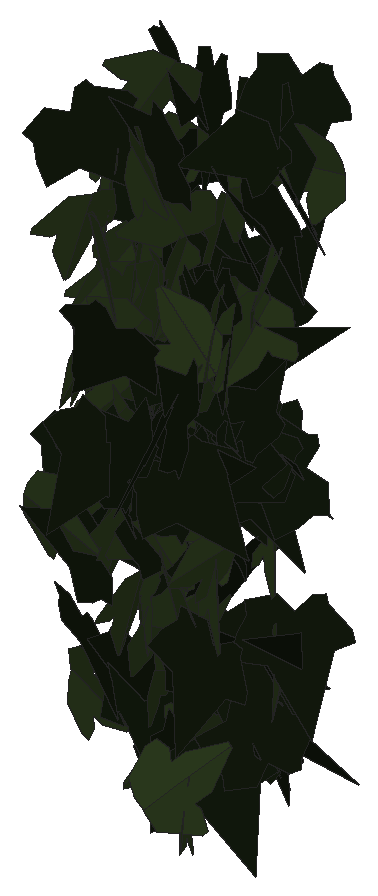
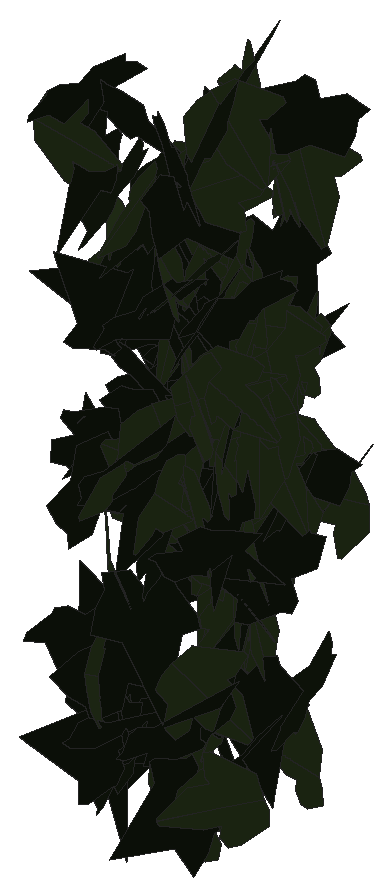
# SketchUp Ruby script. Lengths in inches.
U = 1.inch
M = Sketchup.active_model
def pt(a) = Geom::Point3d.new(a.map { |v| v * U })
def face(e, loops, mat)
  f = e.add_face(loops[0].map { |a| pt(a) })
  loops[1..].each { |l| e.add_face(l.map { |a| pt(a) }).erase! }
  f.material = f.back_material = mat if mat
  f
end
# faces: each face lists its corners as indices into pts; further lists are holes
def faces(e, pts, list, mat = nil) = list.each { |f| face(e, (f[0].is_a?(Array) ? f : [f]).map { |l| l.map { |i| pts[i] } }, mat) }
# xy, xz, yz: faces in a plane at the given z, y or x. An outline is a flat list of corners, or four numbers for a rectangle; further outlines are holes
def ring(l) = l.size == 4 ? [[l[0], l[1]], [l[2], l[1]], [l[2], l[3]], [l[0], l[3]]] : l.each_slice(2).to_a
def flat(e, list, mat, &to3) = list.each { |f| face(e, (f[0].is_a?(Array) ? f : [f]).map { |l| ring(l).map { |u, v| to3.(u, v) } }, mat) }
def xy(e, z, list, mat = nil) = flat(e, list, mat) { |x, y| [x, y, z] }
def xz(e, y, list, mat = nil) = flat(e, list, mat) { |x, z| [x, y, z] }
def yz(e, x, list, mat = nil) = flat(e, list, mat) { |y, z| [x, y, z] }
def lines(e, pts, list) = list.each { |a, b| e.add_line(pt(pts[a]), pt(pts[b])) }
# prism: a flat outline (further loops are holes) pulled along v
def prism(e, loops, v, mat = nil)
  f = face(e, loops, mat); d = Geom::Vector3d.new(v.map { |x| x * U })
  f.pushpull(f.normal.samedirection?(d) ? d.length : -d.length)
end
def box(e, o, s, mat = nil) = prism(e, [[o, [o[0] + s[0], o[1], o[2]], [o[0] + s[0], o[1] + s[1], o[2]], [o[0], o[1] + s[1], o[2]]]], [0, 0, s[2]], mat)
def at(x, y, z, deg = 0) = Geom::Transformation.translation(pt([x, y, z])) * Geom::Transformation.rotation(ORIGIN, Z_AXIS, deg.degrees)
def axes(o, x, y, z) = Geom::Transformation.new([*x, 0, *y, 0, *z, 0, *pt(o).to_a, 1])
def part(name) = M.definitions.add(name)
# library, detail: a bought-in or finely detailed component or shape, given as its bounding box
def library(name, o, s) = part(name).tap { |d| box(d.entities, o, s) }
def detail(e, o, s) = box(e.add_group.entities, o, s)
def put(e, d, t, mat = nil) = e.add_instance(d, t).tap { |i| i.material = mat if mat }
def group(e, t, mat = nil) = e.add_group.tap { |g| g.transformation = t; g.material = mat if mat }.entities
root = M.entities
M.materials.add("efeu1").color = [18, 25, 13]
M.materials.add("efeu2").color = [43, 57, 29]
c1 = part("ivyleaf_10")
p = [[0,0.5,-0.03],[-0.0625,2.02,-0.43],[-0.19,2.01,-0.46],[-0.54,1.05,-0.29],[-0.52,0.625,-0.18],[-0.83,0.76,-0.28],
  [-1.16,0.64,-0.33],[-1.15,0.33,-0.24],[-0.77,-0.39,0.02],[-0.3,-0.51,0.16],[0.04,-0.48,0.23],[-0.02,2.01,-0.4375],
  [-0.06,2.01,-0.43],[0.04,-0.49,0.23],[0.67,-0.49,0.14],[1.38,0.36,-0.2],[1.375,0.51,-0.24],[0.81,0.65,-0.19],
  [0.62,0.59,-0.15],[0.6,1.09,-0.28],[0.5,1.23,-0.31]]
faces(c1.entities,p,[[0,1,2,3,4,5,6,7,8,9,10],[11,12,0,13,14,15,16,17,18,19,20]],"efeu2")
c2 = part("ivyleaf_9")
p = [[1.54,2.16,1.25],[1.36,2.04,1.19],[-0.21,0.99,0.68],[-0.71,1.11,0.82],[-0.85,0.86,0.67],[-0.8,0.17,0.21],
  [-0.9,-0.01,0.1],[-0.67,-0.16,-0.02],[-0.08,-0.08,-0.05],[-0.03,-0.6,-0.4],[0.65,-0.88,-0.66],[0.83,-0.6,-0.49],
  [1.29,-0.42,-0.43],[1.8125,-0.07,-0.26],[1.21,0.44,0.15]]
faces(c2.entities,p,[[0,1,2,3,4,5,6,7,8,9,10,11,12,13,14]],"efeu1")
put(root,c1,axes([29.63,222.12,219.35],[-0.26898,0.10914,-0.40711],[0.32327,-0.25646,-0.28235],[-0.27045,-0.41511,0.0674]))
put(root,c1,axes([30.23,221.64,218.46],[-0.36147,-0.05554,0.34097],[-0.33899,-0.03802,-0.36557],[0.06653,-0.49545,-0.01017]))
put(root,c1,axes([30.02,221.95,220.1],[-0.21554,-0.44343,0.08317],[-0.02161,-0.08192,-0.49277],[0.45064,-0.21602,0.01615]))
put(root,c2,axes([29.64,221.65,215.46],[0.22446,-0.38681,0.2236],[0.09963,-0.20059,-0.44703],[0.43554,0.24524,-0.01298]))
put(root,c1,axes([30,222.03,220.38],[0.07333,0.24047,-0.4322],[-0.16199,-0.40115,-0.25068],[-0.46731,0.17679,0.01908]))
put(root,c1,axes([29.57,221.67,214.59],[0.03065,-0.04016,0.49744],[0.49615,-0.05127,-0.03471],[0.0538,0.49574,0.03671]))
put(root,c1,axes([30.24,222.63,219.8125],[0.27612,0.06542,-0.41168],[-0.41684,0.04646,-0.27219],[0.00264,0.49352,0.08019]))
put(root,c2,axes([29.82,222.73,221.03],[-0.04323,-0.48304,-0.12167],[0.01583,0.12073,-0.48495],[0.49788,-0.04578,0.00485]))
put(root,c1,axes([30.1,221.95,218.91],[-0.34806,-0.35895,0.00311],[-0.00149,-0.00289,-0.49999],[0.35896,-0.34806,0.00094]))
put(root,c1,axes([30.17,221.73,218.73],[-0.01748,-0.22838,0.44445],[-0.04716,-0.44199,-0.22896],[0.49746,-0.04992,-0.00609]))
put(root,c1,axes([30.33,222.75,219.53],[0.01714,0.13451,0.48126],[-0.20471,-0.4374,0.12954],[0.45585,-0.20148,0.04007]))
put(root,c1,axes([30.24,222.03,220.47],[-0.45318,0.19204,0.08801],[-0.07981,0.03721,-0.49218],[-0.19559,-0.46015,-0.00308]))
put(root,c1,axes([29.82,220.66,217.52],[-0.12335,0.05379,-0.48155],[0.44157,-0.19212,-0.13456],[-0.19951,-0.45847,-0.00011]))
put(root,c2,axes([29.91,221.32,218.38],[0.00236,-0.24218,-0.43743],[0.18486,0.40686,-0.22426],[0.46457,-0.16067,0.09145]))
put(root,c2,axes([30.36,222.92,217.68],[-0.38535,-0.27616,0.15887],[-0.1233,-0.10063,-0.47399],[0.29377,-0.40449,0.00945]))
put(root,c1,axes([30.05,222.625,218.82],[0.13286,-0.31833,0.36196],[0.24291,-0.28008,-0.33548],[0.41634,0.26499,0.08023]))
put(root,c2,axes([30.31,222.17,219.47],[0.29122,-0.07064,-0.40025],[-0.38944,0.0924,-0.29966],[0.1163,0.48628,-0.0012]))
put(root,c2,axes([29.97,221.62,216.92],[0.08087,0.03347,0.49228],[0.45491,0.18814,-0.08753],[-0.19109,0.46204,-0.00002]))
put(root,c1,axes([30.29,221.73,217.45],[0.13576,-0.4812,0.00356],[0.00097,-0.00342,-0.49999],[0.48121,0.13577,0]))
put(root,c1,axes([30.08,221.4375,217.75],[-0.20876,-0.15927,-0.4255],[0.3328,0.26517,-0.26254],[0.30929,-0.39283,-0.0047]))
put(root,c1,axes([30.55,221.54,219.77],[-0.36925,-0.1456,0.30406],[-0.27135,-0.13924,-0.39621],[0.20005,-0.45761,0.02381]))
put(root,c1,axes([30.11,221.11,219.5],[0.0309,-0.05768,0.4957],[0.28165,-0.40798,-0.06503],[0.41197,0.28325,0.00728]))
put(root,c2,axes([30.07,220.95,222.72],[0.01722,-0.20561,-0.45544],[0.107,0.44666,-0.19759],[0.48811,-0.09066,0.05939]))
put(root,c2,axes([30.34,221,216.88],[0.15048,-0.47353,-0.05592],[0.0275,-0.04993,0.49674],[-0.47603,-0.15257,0.01102]))
put(root,c2,axes([30.15,223,220.64],[0.01103,-0.39511,0.30622],[-0.00501,-0.30636,-0.39512],[0.49985,0.00565,-0.01072]))
put(root,c1,axes([29.98,222.39,214.33],[0.11317,0.08031,0.48036],[0.34727,0.33246,-0.13739],[-0.34146,0.36472,0.01947]))
put(root,c2,axes([30,221.53,217.92],[0.20469,-0.34611,0.29718],[0.13944,-0.26267,-0.40195],[0.43435,0.24742,-0.01101]))
put(root,c1,axes([30.15,221.52,222.07],[0.34931,-0.26102,0.24465],[0.20487,-0.13436,-0.43586],[0.29328,0.40474,0.01309]))
put(root,c1,axes([30.52,222.1,222.94],[-0.28599,-0.32336,0.25228],[-0.16848,-0.18778,-0.43168],[0.37393,-0.33192,-0.00155]))
put(root,c2,axes([30.44,222.08,218.18],[0.33035,0.04369,-0.37277],[-0.37394,-0.00436,-0.33189],[-0.03226,0.49807,0.0298]))
put(root,c1,axes([30.42,220.72,221.69],[-0.11695,-0.47986,0.07786],[-0.01615,-0.0762,-0.4939],[0.48586,-0.11804,0.00232]))
put(root,c1,axes([30.6,222.6,215.77],[-0.21113,-0.28887,0.34926],[-0.20553,-0.28238,-0.3578],[0.40396,-0.29465,0.00049]))
put(root,c2,axes([30.52,221.61,215.38],[0.25137,0.25331,-0.35022],[-0.25309,-0.24215,-0.3568],[-0.35037,0.35665,0.00648]))
put(root,c1,axes([30.31,222.7,219.15],[0.32938,-0.37434,-0.03713],[0.02483,-0.02761,0.49862],[-0.37536,-0.33031,0.0004]))
put(root,c1,axes([30.44,221.42,217.2],[0.05093,-0.47747,0.13939],[0.02894,-0.13703,-0.47998],[0.49656,0.05696,0.01368]))
put(root,c1,axes([30.75,222.13,221.93],[-0.15932,-0.04876,-0.47142],[-0.43701,-0.17736,0.16604],[-0.18342,0.46493,0.0139]))
put(root,c1,axes([30.41,221.96,220.99],[-0.06647,0.36301,-0.33736],[0.0188,-0.33828,-0.36771],[-0.49521,-0.06156,0.03132]))
put(root,c2,axes([30.3,222,214.65],[0.1057,-0.48864,-0.00758],[-0.00159,0.00741,-0.49994],[0.4887,0.10571,0.00002]))
put(root,c1,axes([30.57,221.47,216.35],[0.05701,-0.49648,0.0162],[0.00135,-0.01615,-0.49974],[0.49674,0.05702,-0.0005]))
put(root,c2,axes([30.34,222.64,222.69],[0.03214,-0.28726,0.40798],[0.11451,-0.39367,-0.2862],[0.48565,0.11183,0.04048]))
put(root,c2,axes([30.68,222.25,215.22],[0.27303,-0.35536,0.22176],[-0.12425,0.18408,0.44797],[-0.40002,-0.29972,0.01221]))
put(root,c1,axes([30.52,221.57,220.01],[-0.45121,0.02215,0.21428],[0.21421,-0.00661,0.45174],[0.02284,0.49947,-0.00352]))
put(root,c1,axes([30.74,222.33,213.88],[0.00643,-0.08137,0.49329],[-0.0088,-0.49328,-0.08125],[0.49988,-0.00764,-0.00777]))
put(root,c1,axes([30.81,222.3,218.07],[0.32473,-0.29879,-0.2351],[-0.1473,0.18616,-0.44005],[0.3505,0.35506,0.03289]))
put(root,c1,axes([30.77,221.64,215.21],[0.0811,-0.22392,-0.43964],[-0.03764,0.44143,-0.23178],[0.49194,0.07069,0.05475]))
put(root,c2,axes([30.96,222.8,214.84],[-0.25328,-0.4306,-0.02069],[-0.00709,-0.01983,0.49956],[-0.43104,0.25335,0.00394]))
put(root,c1,axes([30.625,222.51,219.55],[0.34826,-0.30325,0.1917],[0.14008,-0.13103,-0.46175],[0.33029,0.37532,-0.00631]))
put(root,c2,axes([31.1,221.75,217.01],[-0.35783,0.30321,0.17327],[-0.13687,0.10647,-0.46897],[-0.32129,-0.38305,0.00681]))
put(root,c2,axes([30.89,221.57,217.01],[-0.10067,-0.41188,0.26498],[0.0895,0.2505,0.42337],[-0.48151,0.13267,0.02329]))
put(root,c2,axes([30.81,222.27,214.08],[-0.08691,0.20281,-0.44868],[-0.19267,0.40528,0.22051],[0.45313,0.21123,0.00771]))
put(root,c2,axes([30.89,222.3,222],[-0.10705,0.27082,-0.40644],[0.12755,-0.38615,-0.29089],[-0.47146,-0.16596,0.01358]))
put(root,c2,axes([30.69,222.79,222.7],[-0.29721,0.032,-0.4008],[0.40021,-0.02446,-0.29872],[-0.03873,-0.49837,-0.01107]))
put(root,c1,axes([30.6,221.6,216.21],[-0.14395,0.07829,-0.47239],[0.23124,-0.42057,-0.14017],[-0.41929,-0.25883,0.08488]))
put(root,c1,axes([30.8,222.87,218.21],[0.01492,0.34245,-0.36401],[-0.04068,-0.36213,-0.34235],[-0.49812,0.03983,0.01706]))
put(root,c1,axes([30.74,220.56,221.52],[-0.28518,0.36031,-0.19711],[0.115,-0.16032,-0.45943],[-0.39427,-0.30737,0.00856]))
put(root,c2,axes([31.09,220.43,220.4],[0.20155,0.15169,-0.4317],[-0.34913,-0.25394,-0.25223],[-0.29578,0.40312,0.00356]))
put(root,c1,axes([30.86,221.42,215.95],[-0.08411,-0.26349,-0.41653],[0.1266,0.39682,-0.27659],[0.47634,-0.15199,-0.00004]))
put(root,c2,axes([30.73,222.51,220.8],[-0.05341,-0.44512,0.2214],[0.09503,-0.22771,-0.43488],[0.48797,-0.00437,0.10892]))
put(root,c1,axes([30.95,221.36,217.26],[-0.38009,-0.26991,-0.18079],[0.14404,0.10939,-0.46614],[0.29118,-0.40643,-0.0054]))
put(root,c2,axes([30.87,222.8,218.65],[-0.05364,-0.4957,0.03742],[-0.00261,-0.03735,-0.4986],[0.49711,-0.05369,0.00142]))
put(root,c1,axes([31.22,221.99,217.15],[0.34155,0.0461,-0.36224],[-0.35978,-0.04234,-0.34462],[-0.06245,0.49607,0.00425]))
put(root,c1,axes([31.19,222.39,218.76],[-0.35266,-0.29605,0.1949],[-0.15048,-0.12389,-0.46044],[0.32092,-0.38342,-0.00172]))
put(root,c2,axes([30.97,220.36,218.86],[-0.1254,-0.4109,0.2558],[-0.07934,-0.24322,-0.42959],[0.47747,-0.14833,-0.0042]))
put(root,c1,axes([31.04,222.375,214.55],[0.0025,-0.31291,0.38998],[0.04607,-0.38818,-0.31176],[0.49787,0.03749,0.02689]))
put(root,c2,axes([31.38,221.12,214.27],[-0.14188,0.03076,-0.47846],[-0.47591,0.05146,0.14443],[0.05813,0.49639,0.01468]))
put(root,c2,axes([30.93,221.39,218.8],[-0.03347,0.48146,0.13067],[0.00662,-0.13053,0.48262],[0.49883,0.03404,0.00236]))
put(root,c1,axes([31.2,221.49,221.43],[-0.36094,-0.26885,-0.21782],[-0.17553,-0.12899,0.45006],[-0.29819,0.40135,-0.00127]))
put(root,c2,axes([31.14,221.5,222.23],[0.17695,-0.46656,0.03185],[0.00456,0.03577,0.4987],[-0.46762,-0.1762,0.01692]))
put(root,c1,axes([30.99,222.5,221.01],[0.22723,-0.33331,0.29541],[0.1809,-0.23398,-0.40315],[0.40699,0.29009,0.01426]))
put(root,c1,axes([31.19,221.4,216.6],[-0.40291,0.27624,0.10655],[-0.09027,0.05677,-0.4885],[-0.28198,-0.41288,0.00413]))
put(root,c1,axes([31.11,221.71,220.8],[-0.05545,0.33604,-0.36607],[-0.02637,-0.36981,-0.33548],[-0.49622,-0.0179,0.05874]))
put(root,c2,axes([31.32,222.45,216.55],[-0.02367,0.49172,-0.0875],[-0.00559,-0.08785,-0.49219],[-0.49941,-0.02232,0.00965]))
put(root,c2,axes([31.1,222.89,220.51],[-0.1281,-0.47762,0.07396],[-0.01726,-0.07194,-0.4945],[0.483,-0.12924,0.00194]))
put(root,c2,axes([31.04,222.38,218.04],[0.00803,-0.35271,-0.35431],[-0.0159,0.35399,-0.35275],[0.49968,0.01693,-0.00553]))
put(root,c2,axes([31.61,221.24,218.08],[-0.33515,0.00332,-0.37103],[-0.37104,-0.00618,0.3351],[-0.00236,0.49995,0.00661]))
put(root,c2,axes([31.61,220.11,218.8],[-0.1336,0.1951,0.44055],[-0.24253,0.3678,-0.23643],[-0.41633,-0.27687,-0.00364]))
put(root,c2,axes([31.36,222.36,216.88],[0.17252,-0.40757,0.23264],[-0.03818,0.23485,0.43976],[-0.46774,-0.1695,0.04991]))
put(root,c1,axes([30.95,220.99,222.39],[0.06263,-0.05755,0.49271],[0.47427,-0.13864,-0.07648],[0.14543,0.47693,0.03722]))
put(root,c2,axes([31.04,221.5,219.69],[-0.09699,-0.16118,-0.46327],[0.32781,0.32998,-0.18343],[0.36487,-0.33931,0.04166]))
put(root,c2,axes([31.62,222.67,217.92],[-0.28238,-0.40005,0.10109],[0.05623,0.08404,0.48967],[-0.40878,0.28791,-0.00247]))
put(root,c1,axes([31.4,222.72,218.23],[0.13131,0.44538,-0.18546],[-0.04915,-0.17885,-0.46432],[-0.47994,0.14017,-0.00319]))
put(root,c1,axes([31.42,222.31,221.66],[0.07751,-0.1876,-0.45694],[0.07706,0.46147,-0.17638],[0.48791,-0.04308,0.10045]))
put(root,c2,axes([31.27,222.28,221.7],[0.4461,-0.17322,-0.14488],[-0.12706,0.07266,-0.4781],[0.18668,0.46337,0.02081]))
put(root,c2,axes([31.37,221.58,220.54],[-0.29855,-0.06966,-0.39499],[0.38882,0.07058,-0.30633],[0.09844,-0.49007,0.01203]))
put(root,c2,axes([31.78,222.29,219.44],[-0.4904,0.04818,-0.08475],[0.08492,-0.00239,-0.49273],[-0.04789,-0.49767,-0.00584]))
put(root,c2,axes([31.95,222.51,214.41],[-0.32066,-0.35767,-0.13874],[-0.09512,-0.10105,0.48036],[-0.37166,0.33446,-0.00324]))
put(root,c2,axes([31.43,222.62,220.33],[-0.00033,-0.14815,0.47755],[0.19446,-0.43999,-0.13637],[0.46063,0.18564,0.05791]))
put(root,c2,axes([32.05,222.22,222.59],[-0.44836,0.11725,0.18767],[-0.17757,0.06242,-0.46322],[-0.13206,-0.48203,-0.01434]))
put(root,c1,axes([31.74,221.3,219.71],[-0.02621,-0.41363,-0.27968],[0.02936,0.27831,-0.41435],[0.49845,-0.03815,0.0097]))
put(root,c1,axes([31.82,221.2,219.98],[0.26116,0.36611,0.21853],[-0.12963,-0.17596,0.4497],[0.40619,-0.29154,0.00301]))
put(root,c2,axes([31.93,222.32,214.49],[0.18443,0.00386,-0.46473],[-0.46474,0.00075,-0.18443],[-0.00073,0.49998,0.00386]))
put(root,c1,axes([31.63,221.88,217.89],[0.13506,0.25398,-0.40896],[0.16543,0.3744,0.28715],[0.4521,-0.21288,0.0171]))
put(root,c2,axes([31.39,221.18,218.38],[0.0931,-0.0458,0.48912],[0.39993,-0.28203,-0.10253],[0.28529,0.41032,-0.01588]))
put(root,c2,axes([31.65,222.38,219.97],[-0.15268,-0.09794,0.46594],[0.41893,0.20487,0.18034],[-0.22624,0.44546,0.0195]))
put(root,c2,axes([31.99,222.2,218.58],[-0.38143,-0.25178,0.20278],[-0.17543,-0.10222,-0.45692],[0.27154,-0.41971,-0.01036]))
put(root,c1,axes([31.6,221.12,214.02],[-0.04996,0.10809,-0.48561],[0.18867,-0.44748,-0.11901],[-0.46034,-0.19513,0.00392]))
put(root,c1,axes([31.77,221.85,220.4],[-0.00245,0.35354,-0.35355],[-0.0381,-0.35266,-0.35239],[-0.49854,0.02521,0.02867]))
put(root,c2,axes([31.62,222.66,214.15],[-0.07255,-0.1708,0.46429],[0.10924,-0.4632,-0.15333],[0.4825,0.07919,0.10453]))
put(root,c2,axes([31.65,221.63,220.63],[-0.26609,-0.00733,-0.42325],[0.42144,0.04236,-0.26569],[0.03975,-0.49815,-0.01637]))
put(root,c1,axes([31.57,222.73,217.04],[0.23835,-0.12599,0.42109],[0.35582,-0.2259,-0.269],[0.25803,0.4279,-0.01802]))
put(root,c1,axes([31.71,220.51,214.32],[0.27006,0.07118,-0.41473],[0.26653,0.3524,0.23405],[0.32562,-0.34749,0.15239]))
put(root,c2,axes([31.72,222.14,218.06],[0.24802,-0.38017,-0.20966],[-0.08082,0.19681,-0.45247],[0.42656,0.25834,0.03618]))
put(root,c2,axes([31.86,221.28,216.01],[-0.09379,-0.46842,0.14759],[-0.03032,-0.14445,-0.47772],[0.49019,-0.09856,-0.00131]))
put(root,c2,axes([31.72,222.79,217.75],[0.4536,-0.11799,-0.17414],[0.16911,-0.0416,0.46869],[-0.12509,-0.4841,0.00217]))
put(root,c2,axes([31.85,221.42,214.47],[-0.02097,-0.41604,-0.27653],[0.02342,0.27565,-0.4165],[0.49901,-0.03042,0.00793]))
put(root,c2,axes([31.87,221.47,218.53],[0.06272,-0.07155,-0.49086],[-0.04307,0.49212,-0.07724],[0.49418,0.05197,0.05557]))
put(root,c2,axes([31.73,222.3125,215.29],[0.48634,0.09888,-0.06079],[0.05889,0.01546,0.49628],[0.10003,-0.48988,0.0034]))
put(root,c1,axes([31.98,221.3,217.39],[-0.01122,0.02088,0.49944],[0.13829,-0.47994,0.02317],[0.48036,0.13866,0.00499]))
put(root,c2,axes([31.76,222.44,221.59],[0.23955,-0.41976,0.12813],[0.05693,-0.11501,-0.48325],[0.43517,0.24611,-0.00731]))
put(root,c1,axes([32.2,221.77,220.625],[0.20033,-0.06648,0.45326],[-0.30431,0.35048,0.18591],[-0.34243,-0.35035,0.09996]))
put(root,c2,axes([32.39,222.32,218.18],[-0.12662,-0.16872,-0.45332],[-0.28828,-0.34996,0.21077],[-0.38841,0.31475,-0.00865]))
put(root,c1,axes([31.86,222.72,215.45],[0.10556,-0.20834,0.4421],[0.29341,-0.3347,-0.22779],[0.39085,0.30752,0.05159]))
put(root,c2,axes([31.91,220.61,218.75],[0.00921,-0.27104,-0.42006],[0.01132,0.42014,-0.27085],[0.49979,-0.00452,0.01387]))
put(root,c2,axes([32.0625,221.65,218.83],[-0.33374,0.32702,0.17799],[0.13289,-0.11866,0.46718],[0.34779,0.35914,-0.00771]))
put(root,c2,axes([31.71,222.55,214.48],[0.34254,-0.1872,0.31245],[0.27197,-0.15384,-0.39034],[0.24228,0.43737,-0.00356]))
put(root,c2,axes([32.24,219.98,219.86],[-0.33446,0.26206,-0.26355],[0.20996,-0.15933,-0.42489],[-0.30667,-0.39489,-0.00346]))
put(root,c2,axes([32.02,222.77,223.07],[-0.07736,-0.48991,-0.06328],[0.01644,0.06146,-0.49594],[0.49371,-0.07881,0.0066]))
put(root,c2,axes([32.11,222.26,222.09],[0.41908,-0.06242,-0.26547],[-0.26121,0.04796,-0.42364],[0.07835,0.49376,0.00759]))
put(root,c2,axes([32.31,221.76,214.5],[-0.36025,-0.27905,0.20578],[0.16273,0.12596,0.45569],[-0.30616,0.3953,0.00006]))
put(root,c1,axes([32.24,221.76,220.41],[0.1799,0.34971,-0.30877],[-0.16643,-0.26105,-0.39263],[-0.43582,0.24404,0.02248]))
put(root,c2,axes([31.87,221.65,219.74],[0.13784,0.01253,0.48046],[0.47014,0.1003,-0.1375],[-0.09983,0.48968,0.01587]))
put(root,c1,axes([31.99,221.12,217.19],[0.25361,-0.20239,0.38043],[0.33916,-0.17854,-0.32108],[0.26581,0.42091,0.04673]))
put(root,c1,axes([32.61,222.49,222.19],[0.09189,-0.03046,-0.49054],[-0.4697,0.14148,-0.09677],[0.1447,0.4786,-0.00261]))
put(root,c2,axes([32.15,222.5,216.01],[-0.14844,-0.41079,-0.24335],[0.06963,0.23349,-0.43662],[0.47235,-0.16351,-0.01211]))
put(root,c2,axes([32.64,219.84,219.95],[-0.24962,0.10582,-0.42011],[-0.41946,0.06226,0.26491],[0.10837,0.48469,0.05769]))
